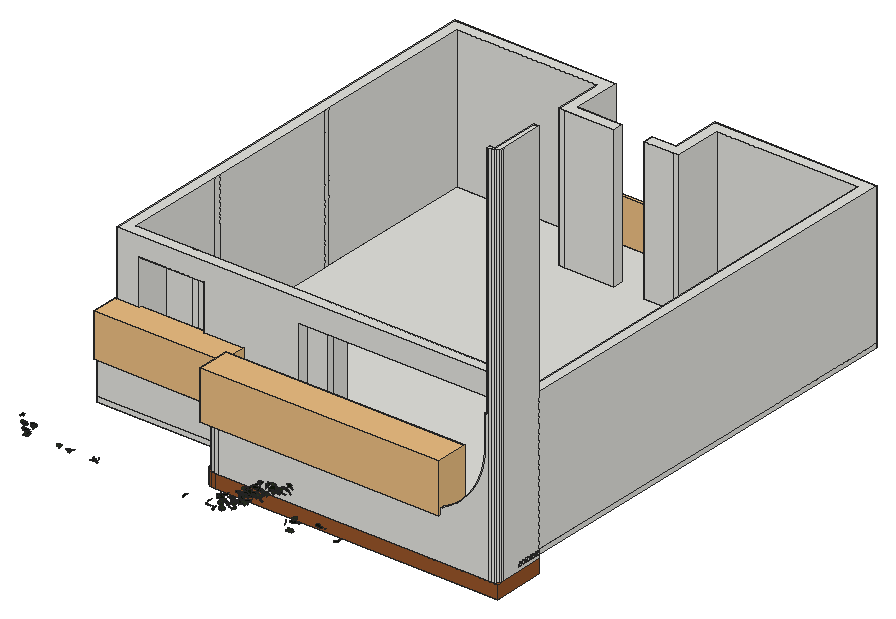
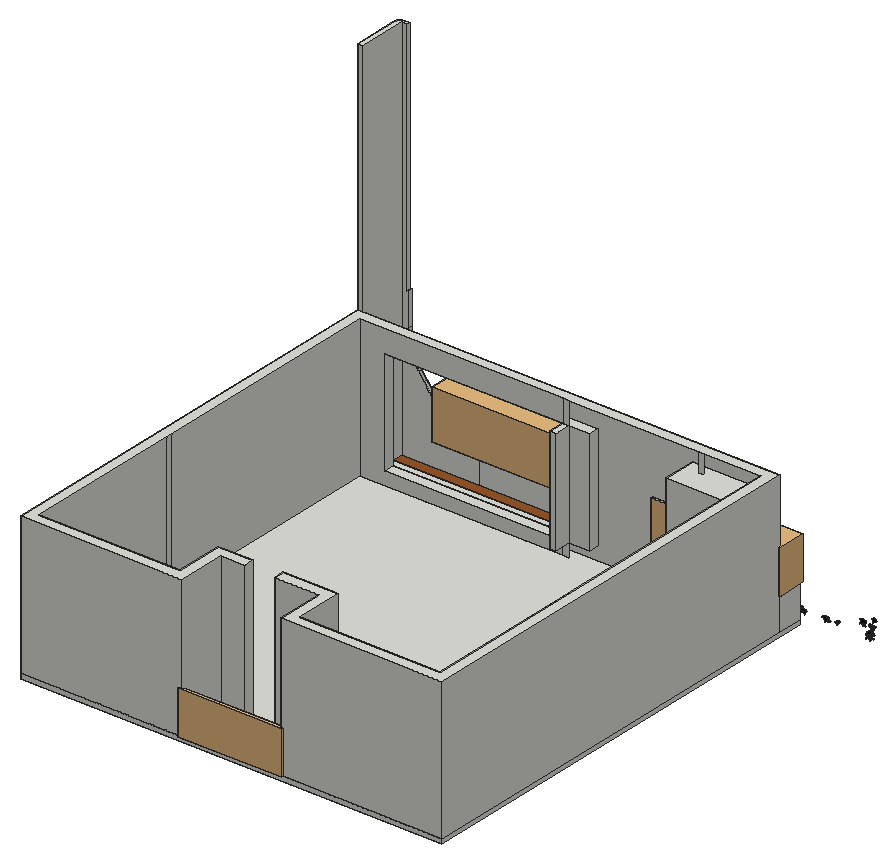
# SketchUp Ruby script. Lengths in millimetres.
U = 1.mm
M = Sketchup.active_model
def pt(a) = Geom::Point3d.new(a.map { |v| v * U })
def face(e, loops, mat)
  f = e.add_face(loops[0].map { |a| pt(a) })
  loops[1..].each { |l| e.add_face(l.map { |a| pt(a) }).erase! }
  f.material = f.back_material = mat if mat
  f
end
# faces: each face lists its corners as indices into pts; further lists are holes
def faces(e, pts, list, mat = nil) = list.each { |f| face(e, (f[0].is_a?(Array) ? f : [f]).map { |l| l.map { |i| pts[i] } }, mat) }
# xy, xz, yz: faces in a plane at the given z, y or x. An outline is a flat list of corners, or four numbers for a rectangle; further outlines are holes
def ring(l) = l.size == 4 ? [[l[0], l[1]], [l[2], l[1]], [l[2], l[3]], [l[0], l[3]]] : l.each_slice(2).to_a
def flat(e, list, mat, &to3) = list.each { |f| face(e, (f[0].is_a?(Array) ? f : [f]).map { |l| ring(l).map { |u, v| to3.(u, v) } }, mat) }
def xy(e, z, list, mat = nil) = flat(e, list, mat) { |x, y| [x, y, z] }
def xz(e, y, list, mat = nil) = flat(e, list, mat) { |x, z| [x, y, z] }
def yz(e, x, list, mat = nil) = flat(e, list, mat) { |y, z| [x, y, z] }
def lines(e, pts, list) = list.each { |a, b| e.add_line(pt(pts[a]), pt(pts[b])) }
# prism: a flat outline (further loops are holes) pulled along v
def prism(e, loops, v, mat = nil)
  f = face(e, loops, mat); d = Geom::Vector3d.new(v.map { |x| x * U })
  f.pushpull(f.normal.samedirection?(d) ? d.length : -d.length)
end
def box(e, o, s, mat = nil) = prism(e, [[o, [o[0] + s[0], o[1], o[2]], [o[0] + s[0], o[1] + s[1], o[2]], [o[0], o[1] + s[1], o[2]]]], [0, 0, s[2]], mat)
def at(x, y, z, deg = 0) = Geom::Transformation.translation(pt([x, y, z])) * Geom::Transformation.rotation(ORIGIN, Z_AXIS, deg.degrees)
def axes(o, x, y, z) = Geom::Transformation.new([*x, 0, *y, 0, *z, 0, *pt(o).to_a, 1])
def part(name) = M.definitions.add(name)
# library, detail: a bought-in or finely detailed component or shape, given as its bounding box
def library(name, o, s) = part(name).tap { |d| box(d.entities, o, s) }
def detail(e, o, s) = box(e.add_group.entities, o, s)
def put(e, d, t, mat = nil) = e.add_instance(d, t).tap { |i| i.material = mat if mat }
def group(e, t, mat = nil) = e.add_group.tap { |g| g.transformation = t; g.material = mat if mat }.entities
root = M.entities
M.materials.add("Emissive").color = [255, 185, 108]
M.materials.add("[Wood Cherry Original]").color = [152, 86, 42]
M.materials.add("efeu1").color = [18, 25, 13]
M.materials.add("efeu2").color = [43, 57, 29]
c1 = part("ivyleaf_10")
p = [[0,12.8,-0.8],[-1.5,51.3,-10.9],[-4.9,51,-11.6],[-13.6,26.5,-7.3],[-13.2,15.9,-4.6],[-21.1,19.3,-7.2],
  [-29.5,16.3,-8.3],[-29.2,8.3,-6.2],[-19.7,-9.8,0.5],[-7.6,-13,4],[1,-12.2,5.8],[-0.4,51.1,-11.1],
  [-1.5,51.1,-10.9],[1,-12.4,5.9],[16.9,-12.4,3.5],[35.1,9.1,-5.1],[35,12.9,-6.1],[20.5,16.4,-4.9],
  [15.8,15,-3.8],[15.3,27.6,-7.1],[12.8,31.3,-7.8]]
faces(c1.entities,p,[[0,1,2,3,4,5,6,7,8,9,10],[11,12,0,13,14,15,16,17,18,19,20]],"efeu2")
c2 = part("ivyleaf_9")
p = [[39.1,54.8,31.7],[34.5,51.8,30.2],[-5.3,25.2,17.3],[-17.9,28.3,20.9],[-21.6,21.7,17],[-20.2,4.3,5.3],
  [-22.9,-0.3,2.5],[-17.1,-4,-0.6],[-2,-2.1,-1.2],[-0.7,-15.4,-10.1],[16.6,-22.3,-16.7],[21.1,-15.1,-12.5],
  [32.7,-10.7,-11],[46.1,-1.8,-6.6],[30.8,11.2,3.8]]
faces(c2.entities,p,[[0,1,2,3,4,5,6,7,8,9,10,11,12,13,14]],"efeu1")
c3 = library("Group\#17",[0,0,0],[2782,637.9,939.4])
c4 = library("Group\#15",[0,0,0],[5171.1,707.5,1057.5])
c5 = part("Group\#8")
g1 = group(c5.entities,at(0,0,0))
xy(g1,0,[[0,0,0,9144,3500.3,9144,3500.3,8102.6,4459.1,8102.6,4459.1,7874,3276.6,7874,3276.6,8915.4,228.6,8915.4,228.6,228.6,8915.4,228.6,8915.4,8915.4,5867.4,8915.4,5867.4,7874,5119.1,7874,5119.1,8102.6,5638.8,8102.6,5638.8,9144,9144,9144,9144,0]])
xy(g1,288,[[3929.6,0,8374.6,228.6],[4394.2,228.6,4521.2,579.4]])
xy(g1,376.3,[[475.3,0,1877,723.9]])
xy(g1,2564.5,[[3929.6,0,8374.6,228.6],[4394.2,228.6,4521.2,579.4]])
xy(g1,2644.4,[[475.3,0,1877,723.9]])
xy(g1,3048,[[0,0,9144,0,9144,9144,5638.8,9144,5638.8,8102.6,5119.1,8102.6,5119.1,7874,5867.4,7874,5867.4,8915.4,8915.4,8915.4,8915.4,228.6,228.6,228.6,228.6,8915.4,3276.6,8915.4,3276.6,7874,4459.1,7874,4459.1,8102.6,3500.3,8102.6,3500.3,9144,0,9144]])
xz(g1,0,[[[0,0,9144,3048],[3929.6,288,8374.6,2564.5],[475.3,376.3,1877,2644.4]]])
xz(g1,228.6,[[1447.8,0,1574.8,3048],[4394.2,0,4521.2,288],[4521.2,0,4521.2,288,8374.6,288,8374.6,2564.5,4521.2,2564.5,4521.2,3048,8915.4,3048,8915.4,0],[3929.6,288,4394.2,2564.5],[4394.2,2564.5,4521.2,3048]])
xz(g1,579.4,[[4394.2,288,4521.2,2564.5]])
xz(g1,723.9,[[475.3,376.3,1877,2644.4]])
xz(g1,7874,[[3276.6,0,3403.6,3048],[3403.6,0,4459.1,3048],[5119.1,0,5740.4,3048],[5740.4,0,5867.4,3048]])
xz(g1,8102.6,[[3500.3,0,4459.1,3048],[5119.1,0,5638.8,3048]])
xz(g1,8915.4,[[228.6,0,3276.6,3048],[5867.4,0,8915.4,3048]])
xz(g1,9144,[[0,0,3500.3,3048],[5638.8,0,9144,3048]])
yz(g1,0,[[0,0,9144,3048]])
yz(g1,228.6,[[228.6,0,2362.2,3048],[2362.2,0,2489.2,3048],[2489.2,0,5334,3048],[5334,0,5461,3048],[5461,0,8915.4,3048]])
yz(g1,475.3,[[0,376.3,723.9,2644.4]])
yz(g1,1877,[[0,376.3,723.9,2644.4]])
yz(g1,3276.6,[[7874,0,8915.4,3048]])
yz(g1,3500.3,[[8102.6,0,9144,3048]])
yz(g1,3929.6,[[0,288,228.6,2564.5]])
yz(g1,4394.2,[[228.6,288,579.4,2564.5]])
yz(g1,4459.1,[[7874,0,8102.6,3048]])
yz(g1,4521.2,[[228.6,288,579.4,2564.5]])
yz(g1,5119.1,[[7874,0,8102.6,3048]])
yz(g1,5638.8,[[8102.6,0,9144,3048]])
yz(g1,5867.4,[[7874,0,8915.4,3048]])
yz(g1,8374.6,[[0,288,228.6,2564.5]])
yz(g1,8915.4,[[228.6,0,5334,3048],[5334,0,5461,3048],[5461,0,8915.4,3048]])
yz(g1,9144,[[0,0,9144,3048]])
c6 = library("Group\#25",[0,0,0],[2238.5,80,939.4])
p = [[1860.6,2460,2644.4],[3261.9,2460,2644.4],[10529.3,1836.4,3149.6],[10398.2,1836.4,3149.6],[10398.2,2446,3149.6],[10529.3,2446,3149.6]]
lines(root,p,[[0,1],[2,3],[4,5]])
put(root,c1,axes([2242.1,873.4,2679.7],[0.29759,-0.97706,-0.24122],[-0.00358,0.24383,-0.98885],[1.91537,0.15226,0.03563]))
put(root,c1,axes([4967.5,859.2,2851.4],[0.50779,0.74564,0.68177],[-0.36504,0.7297,-0.72299],[-1.8879,0.05946,0.32317]))
put(root,c1,axes([2158.9,869.8,2662.5],[-1.58433,0.57744,0.12979],[-0.21128,0.06767,-1.01309],[-1.1064,-0.83979,0.00761]))
put(root,c2,axes([5728.2,895.5,3110.4],[-0.3541,-0.44322,0.99252],[0.43909,-1.00012,-0.40336],[2.02162,0.13959,0.26145]))
put(root,c2,axes([5469.1,858,3018.6],[1.35654,0.76299,0.25695],[0.31308,0.19791,-1.04402],[-1.49993,0.73136,0.01446]))
put(root,c2,axes([724.9,864.8,2660.9],[0.00599,1.02644,-0.04252],[-0.00314,-0.0425,-1.02645],[-1.25332,0.00501,0.00236]))
put(root,c1,axes([684,878,2636.9],[1.19057,0.38067,-0.02341],[-0.02529,-0.01128,-1.04749],[-0.46461,0.97609,-0.00297]))
put(root,c1,axes([1610.6,870,2612.4],[0.34837,-0.0135,1.0075],[-1.8784,0.20373,0.18204],[-0.38602,-1.00352,0.02341]))
put(root,c1,axes([691.1,871.7,2819.8],[-0.60714,0.25021,-0.8928],[-0.93426,0.46035,0.55588],[0.63775,0.91259,-0.03563]))
put(root,c2,axes([4591,877.2,2635.9],[1.62005,-0.33682,0.41046],[0.77692,-0.08081,-0.91287],[0.64621,0.94156,0.06849]))
put(root,c2,axes([4099,856,2629.3],[0.55858,0.36321,1.03584],[1.02656,0.88612,-0.46354],[-1.81947,0.61146,0.05647]))
put(root,c1,axes([1376.7,875.6,2657.5],[1.27455,0.75499,0.11689],[-0.11631,0.20788,-0.99257],[-1.44935,0.64725,0.18245]))
put(root,c1,axes([595.4,883.2,2836.8],[1.06507,0.56369,-0.10968],[-0.10229,-0.07232,-1.03907],[-0.69309,0.87689,-0.01519]))
put(root,c2,axes([1630.6,865.8,2650.6],[1.18403,0.82066,-0.01773],[-0.22401,0.06716,-1.02102],[-1.54611,0.61874,0.13435]))
put(root,c2,axes([809.8,872.9,2874.2],[1.94041,0.16715,-0.03853],[-0.0612,-0.04191,-1.03253],[-0.32068,1.01942,-0.03613]))
put(root,c2,axes([626.5,868.6,2820.3],[1.01133,0.62198,-0.21562],[-0.30144,-0.0274,-1.02894],[-0.7444,0.85611,0.12372]))
put(root,c2,axes([2122.5,870.6,2617.5],[1.93414,0.05111,0.00473],[-0.01003,0.19729,-0.99823],[-0.09717,0.99693,0.1973]))
put(root,c1,axes([4923.3,889.9,2680.2],[1.09544,0.55557,-0.6352],[-0.98394,-0.37555,-0.79693],[-1.26938,0.77054,0.06957]))
put(root,c2,axes([666.7,888.3,2634.2],[-1.20615,0.2778,-0.01695],[0.00023,-0.06187,-1.02521],[-0.33955,-0.98685,0.05951]))
put(root,c2,axes([583.4,867.1,2972.5],[0.68149,0.89293,0.21313],[0.1496,0.17468,-1.0532],[-1.10994,0.57179,-0.01109]))
put(root,c2,axes([6980,884.2,3058.4],[0.79399,0.16085,-1.15793],[2.00309,0.48349,0.44636],[0.96848,-1.13185,0.02611]))
put(root,c2,axes([2108.7,872.1,2628.9],[0.38033,0.98848,0.13533],[-0.0569,0.14388,-1.00685],[-1.89798,0.19376,0.0573]))
put(root,c2,axes([654.6,871.8,2705.4],[1.00699,0.3655,0.52651],[0.55106,0.27736,-0.90063],[-0.55478,0.93892,0.06109]))
put(root,c2,axes([5332.8,887.7,2945.9],[-0.4729,-0.71957,-0.74613],[0.55117,0.68852,-0.76046],[1.89426,-0.37998,0.035]))
put(root,c1,axes([827.3,880,2813.5],[0.68505,-0.31545,-0.90782],[-1.32482,0.58282,-0.47852],[1.26115,0.7836,-0.00955]))
put(root,c1,axes([614,890.3,2761],[0.32792,-0.99845,-0.0849],[-0.04066,0.07894,-1.03393],[1.22183,0.2706,-0.01162]))
put(root,c1,axes([5409.5,893.3,2948.9],[2.01643,-0.11215,-0.11915],[-0.22506,0.01476,-1.06541],[0.21524,1.06607,0.00222]))
put(root,c2,axes([4719.6,879.5,2604.8],[0.15912,0.02228,-1.00472],[-1.7006,0.46305,-0.06409],[0.87533,0.89557,0.05813]))
put(root,c1,axes([610.5,895.2,2693.7],[-1.21188,-0.22111,0.05207],[-0.05777,-0.02687,-1.01754],[0.27105,-0.99435,0.01591]))
put(root,c1,axes([6293.6,880.7,2880],[0.29531,-0.72314,-1.01067],[-0.35276,0.99366,-0.73943],[2.33871,0.24119,0.01609]))
put(root,c1,axes([4877.8,895.9,2644.8],[1.73286,0.40859,0.19804],[0.28431,0.14949,-0.99524],[-0.81604,0.91972,0.07378]))
put(root,c2,axes([651.5,894.1,2658.9],[1.23921,-0.1475,-0.04468],[-0.05298,0.01185,-1.02638],[0.1804,1.01666,0.00548]))
put(root,c1,axes([686.9,895.7,2656.7],[0.6209,0.83618,0.3194],[0.1711,0.28839,-0.97846],[-1.07854,0.52712,0.02865]))
put(root,c2,axes([711.3,906,2616.1],[-1.11801,0.34409,0.24843],[-0.2952,0.06208,-0.97852],[-0.42538,-0.94745,0.02611]))
put(root,c1,axes([661.3,885.6,2591],[-0.01799,0.45905,-0.93566],[0.02275,0.93572,0.45878],[1.27128,-0.01025,-0.02145]))
put(root,c2,axes([4737.8,890.4,2611.3],[-0.17432,0.95753,0.30224],[-0.07245,0.29996,-0.96186],[-1.90962,-0.09879,0.0089]))
put(root,c1,axes([6459,887,3011.5],[0.43261,0.68832,0.95487],[0.34183,0.94084,-0.72096],[-2.21401,0.27975,0.07527]))
put(root,c2,axes([696.6,888.8,2641.7],[0.73939,0.77669,0.281],[0.16249,0.25207,-0.98399],[-0.99448,0.61865,0.04815]))
put(root,c2,axes([6416,895.1,2928.2],[1.83795,0.2001,0.67518],[1.25058,0.15607,-0.9861],[-0.48199,1.16796,0.01609]))
put(root,c1,axes([5158.9,923.7,2746.8],[0.06803,0.74348,-0.73897],[-1.07018,-0.61042,-0.64135],[-1.68372,0.41802,0.37778]))
put(root,c1,axes([6374,929.2,2723.5],[1.02772,0.08734,-1.12827],[-2.12441,-0.1645,-0.54697],[-0.35423,1.23997,0.00691]))
put(root,c1,axes([626.7,907.5,2629.8],[0.08799,0.56648,0.83577],[-0.5279,0.77439,-0.48754],[-1.11293,-0.32253,0.29733]))
put(root,c2,axes([7360.5,914,2874.3],[0.99165,1.17741,0.39801],[0.30308,0.36477,-1.28755],[-2.34592,0.54483,0.0019]))
put(root,c2,axes([5096.3,1016.4,2816.7],[1.61558,-0.4369,-0.43493],[-0.67908,0.25539,-0.95294],[0.95679,0.91899,0.05806]))
put(root,c2,axes([5354.1,1034.3,3117.3],[-0.98874,-0.36875,-0.89917],[1.67357,0.25577,-0.61295],[0.78754,-1.00647,0.17367]))
put(root,c2,axes([5931.6,1031.2,3365.2],[-1.98819,0.52194,0.01236],[-0.02445,0.00195,-1.16778],[-0.99334,-1.04473,0.004]))
put(root,c2,axes([5387.1,1037,3161.5],[-1.30777,0.56503,-0.61847],[0.72498,-0.50168,-0.88156],[-1.41997,-0.77652,0.11951]))
put(root,c2,axes([5298.2,1018.6,3047.3],[1.5576,0.68968,-0.24282],[-0.37984,-0.1399,-1.07006],[-1.33874,0.84213,0.0211]))
put(root,c2,axes([5616.5,1025,3357.9],[1.76921,-0.04931,0.62228],[1.18679,0.12456,-0.92166],[-0.05451,1.1117,0.13087]))
put(root,c2,axes([5493.5,1032.3,3222],[1.0405,0.65027,-0.69072],[-0.97441,-0.46888,-0.84667],[-1.51996,0.74574,0.06995]))
put(root,c1,axes([5249.1,1042.8,3113.7],[0.64652,1.01263,-0.20331],[-0.17538,-0.18345,-1.06771],[-1.95787,0.35082,0.02851]))
put(root,c1,axes([5602.3,1031,3339],[-0.30681,1.04009,0.36399],[-0.09139,0.36088,-1.05249],[-2.09523,-0.16804,-0.00739]))
put(root,c2,axes([5518.4,1027.3,3267.7],[0.90088,0.98786,0.11357],[0.06997,0.10831,-1.09532],[-1.89118,0.47458,0.01358]))
put(root,c2,axes([4778.7,1052.3,2770.1],[-1.94504,0.12001,0.16733],[-0.3162,0.01988,-1.02901],[-0.23152,-1.0354,-0.00036]))
put(root,c2,axes([5199.6,1054.3,2899.6],[1.00746,-0.95965,0.0234],[0.04472,-0.01376,-1.09588],[1.8264,0.52969,0.01393]))
put(root,c1,axes([5145.5,1048.6,2992.1],[0.69393,0.97253,-0.19472],[-0.23672,-0.16099,-1.03696],[-1.87275,0.38071,0.05892]))
put(root,c1,axes([6035.4,1046.8,3358.8],[-1.56865,-0.81256,-0.11223],[0.195,0.05587,-1.15696],[1.54891,-0.82994,0.03199]))
put(root,c1,axes([6012.2,1053.4,3344.1],[-0.6475,-1.1092,0.03978],[0.68741,-0.14998,-1.09302],[1.9974,-0.30795,0.38906]))
put(root,c1,axes([5732.1,1051.9,3170.1],[2.0977,-0.07402,0.25396],[0.49824,0.14926,-1.0927],[0.07216,1.12118,0.16224]))
put(root,c2,axes([5578.6,1058.5,3196.6],[-1.20779,0.6911,-0.64158],[0.80648,-0.48186,-0.9382],[-1.6033,-0.763,0.01139]))
put(root,c2,axes([4756.1,1049.5,2783.6],[-0.7255,0.91992,-0.26859],[0.15775,-0.25632,-0.99556],[-1.81705,-0.38955,0.02081]))
put(root,c1,axes([5905.9,1055.8,3388.3],[2.00327,-0.33927,-0.20892],[-0.36497,0.08593,-1.10567],[0.6647,1.06967,0.02256]))
put(root,c1,axes([5654.4,1055.3,3191.2],[1.20275,-0.88658,-0.11473],[0.06846,0.1656,-1.0816],[1.70004,0.62057,0.12472]))
put(root,c1,axes([5579,1056.1,3074.9],[1.98723,-0.0017,0.4011],[0.75385,0.18066,-1.03034],[-0.12031,1.10386,0.16924]))
put(root,c2,axes([4850.7,1051.6,2714.5],[1.25281,0.26493,-0.7795],[-1.39844,-0.26112,-0.70925],[-0.70676,0.98628,0.02161]))
put(root,c2,axes([5115.2,1046.6,2980.6],[1.57089,0.01301,0.69398],[1.26714,0.28996,-0.79731],[-0.37342,1.03866,0.21388]))
put(root,c1,axes([4738.1,1072.3,2657.9],[0.68708,0.55538,-0.76273],[-0.9381,-0.58534,-0.65952],[-1.53116,0.60784,0.06181]))
put(root,c1,axes([5712.2,1063.4,3165.4],[-0.17705,-1.12959,-0.04249],[0.05199,0.04038,-1.13316],[2.15072,-0.09397,0.02389]))
put(root,c1,axes([5241.4,1067.2,2980.7],[-1.50802,0.42248,-0.63949],[0.9626,-0.40287,-0.89284],[-1.096,-0.93514,0.09573]))
put(root,c1,axes([5271.5,1068.8,2956.3],[-0.01799,-1.05869,0.08056],[0.05869,-0.0808,-1.05826],[2.01987,-0.00708,0.03147]))
put(root,c1,axes([4739.7,1060.1,2618.7],[-1.89903,0.13306,0.2763],[-0.51695,0.05316,-1.00651],[-0.27096,-1.03399,-0.01619]))
put(root,c2,axes([4728.5,1053.6,2761.5],[-0.66833,0.80842,0.52756],[-0.49945,0.4603,-0.88003],[-1.76804,-0.43562,0.04917]))
put(root,c2,axes([4722.9,1058.2,2741.6],[1.38605,0.40307,-0.59217],[-1.12846,-0.13467,-0.82086],[-0.76502,0.92893,0.13795]))
put(root,c1,axes([5935.1,1068.6,3269.4],[1.24034,-0.07385,0.94765],[1.80339,0.14119,-0.64064],[-0.14283,1.14142,0.14056]))
put(root,c2,axes([5275.8,1060.8,2974.8],[1.78278,-0.1931,-0.46559],[-0.83018,0.18181,-0.953],[0.48071,1.03014,0.08091]))
put(root,c2,axes([5166.2,1073.6,2909.5],[0.37753,-0.94925,-0.41107],[0.15478,0.43158,-0.95735],[1.96264,0.14856,0.15457]))
put(root,c2,axes([6152.4,1080.9,3377.4],[1.15246,-0.99144,0.14789],[0.18487,-0.11393,-1.1615],[1.89881,0.61284,0.02332]))
put(root,c2,axes([5310.5,1071.8,3007.9],[-0.15698,-0.22134,-1.041],[1.60289,0.62477,-0.19957],[1.23835,-0.83675,0.12636]))
put(root,c1,axes([5157.7,1074.1,2817.4],[0.90985,-0.96265,-0.08008],[0.31675,0.1701,-1.0512],[1.81095,0.4539,0.22409]))
put(root,c1,axes([5734.3,1069.3,3288.7],[0.59861,-0.97288,-0.4263],[-0.22162,0.41034,-1.02236],[2.00936,0.33509,0.01424]))
put(root,c1,axes([4997.6,1074.3,2770.1],[-0.88592,-0.91247,-0.12137],[0.43309,0.01771,-1.00594],[1.69753,-0.48073,0.19331]))
put(root,c1,axes([4960,1074.4,2816.4],[-1.36327,-0.74428,0.00579],[-0.00611,-0.00494,-1.03298],[1.41655,-0.71631,0.00111]))
put(root,c2,axes([4502.1,1063.3,2600.4],[-0.15659,0.99517,0.0254],[-0.06349,0.02271,-0.99807],[-1.89356,-0.08306,0.03136]))
put(root,c2,axes([5777,1053.6,3338.6],[0.22454,0.63617,0.90572],[-0.36519,0.90882,-0.61334],[-2.07459,-0.09112,0.20599]))
put(root,c1,axes([4973.2,1072.8,2797.9],[0.07438,1.03091,0.06279],[-0.00467,0.06293,-1.03164],[-1.96566,0.03886,0.00483]))
put(root,c2,axes([4823.4,1057.2,2828.6],[1.16542,0.69984,0.47488],[0.46449,0.41513,-0.92648],[-1.54116,0.65433,0.07987]))
put(root,c1,axes([5873.9,1074.8,3257.7],[-1.87612,0.38988,0.45301],[-0.95555,-0.06614,-1.03562],[-0.61712,-1.08286,0.22635]))
put(root,c2,axes([5442,1063.6,3075],[1.76945,0.54423,0.06894],[0.07148,0.07219,-1.07643],[-1.04161,0.92948,0.04324]))
put(root,c2,axes([4854,1076,2639.1],[1.67937,-0.51416,-0.24126],[-0.2851,0.21927,-1.01521],[1.04264,0.88811,0.11099]))
put(root,c1,axes([4978.9,1078.8,2782.2],[-1.47353,0.67422,0.12444],[-0.37453,-0.03873,-1.01453],[-1.24994,-0.78322,0.15729]))
put(root,c1,axes([4992.7,1079.7,2710.3],[-1.80108,0.43212,0.20093],[-0.3777,0.04881,-1.03966],[-0.82458,-0.96621,0.03734]))
put(root,c2,axes([5608.9,1110.8,3107.8],[-0.49555,-0.71974,0.82282],[0.18275,-0.85762,-0.7198],[2.07251,-0.09647,0.26021]))
put(root,c1,axes([5469.8,1086.7,3019.5],[-1.99649,-0.30508,-0.21695],[0.43862,-0.01764,-1.08956],[0.56145,-1.07107,0.07974]))
put(root,c1,axes([5452.7,1094.3,3000.8],[-1.3568,0.81841,-0.22686],[0.27371,-0.17558,-1.08535],[-1.593,-0.72724,0.00674]))
put(root,c1,axes([5053.8,1098.1,2759.4],[1.80273,0.36869,-0.33995],[-0.66553,-0.03519,-1.01251],[-0.68413,1.00575,0.08919]))
put(root,c2,axes([5956.1,1089.7,3255.1],[1.77598,0.05882,0.67245],[1.276,0.05245,-0.93497],[-0.14916,1.14901,0.00825]))
put(root,c1,axes([5183.8,1102.4,2783.9],[1.47497,-0.71395,-0.2171],[-0.34001,0.12638,-1.05337],[1.37893,0.79484,-0.02752]))
put(root,c2,axes([6181.3,1109.2,3466.2],[0.7666,-1.07979,-0.23813],[-0.12373,0.22987,-1.15231],[2.10079,0.40756,0.01903]))
put(root,c2,axes([5815.1,1109.6,3247.7],[-0.46848,-1.0055,-0.48905],[0.22168,0.47498,-1.03519],[2.11643,-0.27232,0.00017]))
put(root,c2,axes([6064.7,1108.1,3368.3],[2.01851,-0.47378,0.069],[0.11377,-0.03535,-1.16157],[0.90407,1.06224,-0.00788]))
put(root,c1,axes([4949.5,1119.2,2688.5],[-1.5966,-0.40827,-0.49554],[1.01279,0.01408,-0.91248],[0.68373,-0.97423,0.19448]))
put(root,c2,axes([4874.9,1132.3,2633.6],[1.63187,0.58964,0.10067],[0.10232,0.09927,-1.03936],[-1.13384,0.8576,0.0511]))
g2 = group(root,at(4151.8,1531.6,2669.4),"[Wood Cherry Original]")
xy(g2,0,[[[6377.5,-209.6,265.9,-209.5,184.6,-202.2,118.2,-180,66.5,-143.1,29.5,-91.4,7.4,-24.9,0,56.3,0,914.4,6377.5,914.4],[4138.7,109.7,4197.4,117.4,4252.2,140.1,4299.2,176.2,4335.3,223.2,4357.9,278,4365.7,336.7,4357.9,395.5,4335.3,450.2,4299.2,497.2,4252.2,533.3,4197.4,556,4138.7,563.7,4079.9,556,4025.1,533.3,3978.1,497.2,3942.1,450.2,3919.4,395.5,3911.6,336.7,3919.4,278,3942.1,223.2,3978.1,176.2,4025.1,140.1,4079.9,117.4],[2346.9,109.7,2405.7,117.4,2460.4,140.1,2507.4,176.2,2543.5,223.2,2566.2,278,2573.9,336.7,2566.2,395.5,2543.5,450.2,2507.4,497.2,2460.4,533.3,2405.7,556,2346.9,563.7,2288.1,556,2233.4,533.3,2186.4,497.2,2150.3,450.2,2127.6,395.5,2119.9,336.7,2127.6,278,2150.3,223.2,2186.4,176.2,2233.4,140.1,2288.1,117.4],[555.1,109.7,613.9,117.4,668.6,140.1,715.7,176.2,751.7,223.2,774.4,278,782.1,336.7,774.4,395.5,751.7,450.2,715.7,497.2,668.6,533.3,613.9,556,555.1,563.7,496.4,556,441.6,533.3,394.6,497.2,358.5,450.2,335.9,395.5,328.1,336.7,335.9,278,358.5,223.2,394.6,176.2,441.6,140.1,496.4,117.4],[5930.4,109.7,5989.2,117.4,6043.9,140.1,6090.9,176.2,6127,223.2,6149.7,278,6157.4,336.7,6149.7,395.5,6127,450.2,6090.9,497.2,6043.9,533.3,5989.2,556,5930.4,563.7,5871.7,556,5816.9,533.3,5769.9,497.2,5733.8,450.2,5711.1,395.5,5703.4,336.7,5711.1,278,5733.8,223.2,5769.9,176.2,5816.9,140.1,5871.7,117.4]],[[555.1,109.7,496.4,117.4,441.6,140.1,394.6,176.2,358.5,223.2,335.9,278,328.1,336.7,335.9,395.5,358.5,450.2,394.6,497.2,441.6,533.3,496.4,556,555.1,563.7,613.9,556,668.6,533.3,715.7,497.2,751.7,450.2,774.4,395.5,782.1,336.7,774.4,278,751.7,223.2,715.7,176.2,668.6,140.1,613.9,117.4],[555.1,166.8,599.1,172.6,640.1,189.6,675.2,216.6,702.2,251.8,719.2,292.7,725,336.7,719.2,380.7,702.2,421.6,675.2,456.8,640.1,483.8,599.1,500.8,555.1,506.6,511.2,500.8,470.2,483.8,435,456.8,408,421.6,391.1,380.7,385.3,336.7,391.1,292.7,408,251.8,435,216.6,470.2,189.6,511.2,172.6]],[[2346.9,109.7,2288.1,117.4,2233.4,140.1,2186.4,176.2,2150.3,223.2,2127.6,278,2119.9,336.7,2127.6,395.5,2150.3,450.2,2186.4,497.2,2233.4,533.3,2288.1,556,2346.9,563.7,2405.7,556,2460.4,533.3,2507.4,497.2,2543.5,450.2,2566.2,395.5,2573.9,336.7,2566.2,278,2543.5,223.2,2507.4,176.2,2460.4,140.1,2405.7,117.4],[2346.9,166.8,2390.9,172.6,2431.8,189.6,2467,216.6,2494,251.8,2511,292.7,2516.8,336.7,2511,380.7,2494,421.6,2467,456.8,2431.8,483.8,2390.9,500.8,2346.9,506.6,2302.9,500.8,2262,483.8,2226.8,456.8,2199.8,421.6,2182.8,380.7,2177,336.7,2182.8,292.7,2199.8,251.8,2226.8,216.6,2262,189.6,2302.9,172.6]],[[4138.7,109.7,4079.9,117.4,4025.1,140.1,3978.1,176.2,3942.1,223.2,3919.4,278,3911.6,336.7,3919.4,395.5,3942.1,450.2,3978.1,497.2,4025.1,533.3,4079.9,556,4138.7,563.7,4197.4,556,4252.2,533.3,4299.2,497.2,4335.3,450.2,4357.9,395.5,4365.7,336.7,4357.9,278,4335.3,223.2,4299.2,176.2,4252.2,140.1,4197.4,117.4],[4138.7,166.8,4182.6,172.6,4223.6,189.6,4258.8,216.6,4285.8,251.8,4302.7,292.7,4308.5,336.7,4302.7,380.7,4285.8,421.6,4258.8,456.8,4223.6,483.8,4182.6,500.8,4138.7,506.6,4094.7,500.8,4053.7,483.8,4018.5,456.8,3991.5,421.6,3974.6,380.7,3968.8,336.7,3974.6,292.7,3991.5,251.8,4018.5,216.6,4053.7,189.6,4094.7,172.6]],[[5930.4,109.7,5871.7,117.4,5816.9,140.1,5769.9,176.2,5733.8,223.2,5711.1,278,5703.4,336.7,5711.1,395.5,5733.8,450.2,5769.9,497.2,5816.9,533.3,5871.7,556,5930.4,563.7,5989.2,556,6043.9,533.3,6090.9,497.2,6127,450.2,6149.7,395.5,6157.4,336.7,6149.7,278,6127,223.2,6090.9,176.2,6043.9,140.1,5989.2,117.4],[5930.4,166.8,5974.4,172.6,6015.3,189.6,6050.5,216.6,6077.5,251.8,6094.5,292.7,6100.3,336.7,6094.5,380.7,6077.5,421.6,6050.5,456.8,6015.3,483.8,5974.4,500.8,5930.4,506.6,5886.4,500.8,5845.5,483.8,5810.3,456.8,5783.3,421.6,5766.3,380.7,5760.5,336.7,5766.3,292.7,5783.3,251.8,5810.3,216.6,5845.5,189.6,5886.4,172.6]]])
xy(g2,100,[[555.1,166.8,511.2,172.6,470.2,189.6,435,216.6,408,251.8,391.1,292.7,385.3,336.7,391.1,380.7,408,421.6,435,456.8,470.2,483.8,511.2,500.8,555.1,506.6,599.1,500.8,640.1,483.8,675.2,456.8,702.2,421.6,719.2,380.7,725,336.7,719.2,292.7,702.2,251.8,675.2,216.6,640.1,189.6,599.1,172.6]],"Emissive")
xy(g2,138.1,[[2346.9,166.8,2302.9,172.6,2262,189.6,2226.8,216.6,2199.8,251.8,2182.8,292.7,2177,336.7,2182.8,380.7,2199.8,421.6,2226.8,456.8,2262,483.8,2302.9,500.8,2346.9,506.6,2390.9,500.8,2431.8,483.8,2467,456.8,2494,421.6,2511,380.7,2516.8,336.7,2511,292.7,2494,251.8,2467,216.6,2431.8,189.6,2390.9,172.6],[4138.7,166.8,4094.7,172.6,4053.7,189.6,4018.5,216.6,3991.5,251.8,3974.6,292.7,3968.8,336.7,3974.6,380.7,3991.5,421.6,4018.5,456.8,4053.7,483.8,4094.7,500.8,4138.7,506.6,4182.6,500.8,4223.6,483.8,4258.8,456.8,4285.8,421.6,4302.7,380.7,4308.5,336.7,4302.7,292.7,4285.8,251.8,4258.8,216.6,4223.6,189.6,4182.6,172.6],[5930.4,166.8,5886.4,172.6,5845.5,189.6,5810.3,216.6,5783.3,251.8,5766.3,292.7,5760.5,336.7,5766.3,380.7,5783.3,421.6,5810.3,456.8,5845.5,483.8,5886.4,500.8,5930.4,506.6,5974.4,500.8,6015.3,483.8,6050.5,456.8,6077.5,421.6,6094.5,380.7,6100.3,336.7,6094.5,292.7,6077.5,251.8,6050.5,216.6,6015.3,189.6,5974.4,172.6]],"Emissive")
xy(g2,290.5,[[6377.5,-209.6,6377.5,914.4,0,914.4,0,56.3,7.4,-24.9,29.5,-91.4,66.5,-143.1,118.2,-180,184.6,-202.2,265.9,-209.5]])
xz(g2,914.4,[[0,0,6377.5,290.5]])
yz(g2,0,[[56.3,0,914.4,290.5]])
yz(g2,6377.5,[[-209.6,0,914.4,290.5]])
p = [[265.9,-209.5,0],[6377.5,-209.6,0],[6377.5,-209.6,290.5],[265.9,-209.5,290.5],[184.6,-202.2,290.5],[184.6,-202.2,0],
  [118.2,-180,290.5],[118.2,-180,0],[66.5,-143.1,290.5],[66.5,-143.1,0],[29.5,-91.4,290.5],[29.5,-91.4,0],
  [7.4,-24.9,290.5],[7.4,-24.9,0],[0,56.3,290.5],[0,56.3,0],[555.1,166.8,0],[511.2,172.6,0],
  [511.2,172.6,100],[555.1,166.8,100],[599.1,172.6,0],[599.1,172.6,100],[2346.9,166.8,0],[2302.9,172.6,0],
  [2302.9,172.6,138.1],[2346.9,166.8,138.1],[2390.9,172.6,0],[2390.9,172.6,138.1],[4138.7,166.8,0],[4094.7,172.6,0],
  [4094.7,172.6,138.1],[4138.7,166.8,138.1],[4182.6,172.6,0],[4182.6,172.6,138.1],[5930.4,166.8,0],[5886.4,172.6,0],
  [5886.4,172.6,138.1],[5930.4,166.8,138.1],[5974.4,172.6,0],[5974.4,172.6,138.1],[470.2,189.6,0],[470.2,189.6,100],
  [640.1,189.6,0],[640.1,189.6,100],[2262,189.6,0],[2262,189.6,138.1],[2431.8,189.6,0],[2431.8,189.6,138.1],
  [4053.7,189.6,0],[4053.7,189.6,138.1],[4223.6,189.6,0],[4223.6,189.6,138.1],[5845.5,189.6,0],[5845.5,189.6,138.1],
  [6015.3,189.6,0],[6015.3,189.6,138.1],[435,216.6,0],[435,216.6,100],[675.2,216.6,0],[675.2,216.6,100],
  [2226.8,216.6,0],[2226.8,216.6,138.1],[2467,216.6,0],[2467,216.6,138.1],[4018.5,216.6,0],[4018.5,216.6,138.1],
  [4258.8,216.6,0],[4258.8,216.6,138.1],[5810.3,216.6,0],[5810.3,216.6,138.1],[6050.5,216.6,0],[6050.5,216.6,138.1],
  [408,251.8,0],[408,251.8,100],[702.2,251.8,0],[702.2,251.8,100],[2199.8,251.8,0],[2199.8,251.8,138.1],
  [2494,251.8,0],[2494,251.8,138.1],[3991.5,251.8,0],[3991.5,251.8,138.1],[4285.8,251.8,0],[4285.8,251.8,138.1],
  [5783.3,251.8,0],[5783.3,251.8,138.1],[6077.5,251.8,0],[6077.5,251.8,138.1],[391.1,292.7,0],[391.1,292.7,100],
  [719.2,292.7,0],[719.2,292.7,100],[2182.8,292.7,0],[2182.8,292.7,138.1],[2511,292.7,0],[2511,292.7,138.1],
  [3974.6,292.7,0],[3974.6,292.7,138.1],[4302.7,292.7,0],[4302.7,292.7,138.1],[5766.3,292.7,0],[5766.3,292.7,138.1],
  [6094.5,292.7,0],[6094.5,292.7,138.1],[385.3,336.7,0],[385.3,336.7,100],[725,336.7,0],[725,336.7,100],
  [2177,336.7,0],[2177,336.7,138.1],[2516.8,336.7,0],[2516.8,336.7,138.1],[3968.8,336.7,0],[3968.8,336.7,138.1],
  [4308.5,336.7,0],[4308.5,336.7,138.1],[5760.5,336.7,0],[5760.5,336.7,138.1],[6100.3,336.7,0],[6100.3,336.7,138.1],
  [391.1,380.7,0],[391.1,380.7,100],[719.2,380.7,0],[719.2,380.7,100],[2182.8,380.7,0],[2182.8,380.7,138.1],
  [2511,380.7,0],[2511,380.7,138.1],[3974.6,380.7,0],[3974.6,380.7,138.1],[4302.7,380.7,0],[4302.7,380.7,138.1],
  [5766.3,380.7,0],[5766.3,380.7,138.1],[6094.5,380.7,0],[6094.5,380.7,138.1],[408,421.6,0],[408,421.6,100],
  [702.2,421.6,0],[702.2,421.6,100],[2199.8,421.6,0],[2199.8,421.6,138.1],[2494,421.6,0],[2494,421.6,138.1],
  [3991.5,421.6,0],[3991.5,421.6,138.1],[4285.8,421.6,0],[4285.8,421.6,138.1],[5783.3,421.6,0],[5783.3,421.6,138.1],
  [6077.5,421.6,0],[6077.5,421.6,138.1],[435,456.8,0],[435,456.8,100],[675.2,456.8,0],[675.2,456.8,100],
  [2226.8,456.8,0],[2226.8,456.8,138.1],[2467,456.8,0],[2467,456.8,138.1],[4018.5,456.8,0],[4018.5,456.8,138.1],
  [4258.8,456.8,0],[4258.8,456.8,138.1],[5810.3,456.8,0],[5810.3,456.8,138.1],[6050.5,456.8,0],[6050.5,456.8,138.1],
  [470.2,483.8,0],[470.2,483.8,100],[640.1,483.8,0],[640.1,483.8,100],[2262,483.8,0],[2262,483.8,138.1],
  [2431.8,483.8,0],[2431.8,483.8,138.1],[4053.7,483.8,0],[4053.7,483.8,138.1],[4223.6,483.8,0],[4223.6,483.8,138.1],
  [5845.5,483.8,0],[5845.5,483.8,138.1],[6015.3,483.8,0],[6015.3,483.8,138.1],[511.2,500.8,0],[511.2,500.8,100],
  [599.1,500.8,0],[599.1,500.8,100],[2302.9,500.8,0],[2302.9,500.8,138.1],[2390.9,500.8,0],[2390.9,500.8,138.1],
  [4094.7,500.8,0],[4094.7,500.8,138.1],[4182.6,500.8,0],[4182.6,500.8,138.1],[5886.4,500.8,0],[5886.4,500.8,138.1],
  [5974.4,500.8,0],[5974.4,500.8,138.1],[555.1,506.6,0],[555.1,506.6,100],[2346.9,506.6,0],[2346.9,506.6,138.1],
  [4138.7,506.6,0],[4138.7,506.6,138.1],[5930.4,506.6,0],[5930.4,506.6,138.1]]
faces(g2,p,[[0,1,2,3],[0,3,4,5],[5,4,6,7],[7,6,8,9],[9,8,10,11],[11,10,12,13],[13,12,14,15]])
faces(g2,p,[[16,17,18,19],[20,16,19,21],[22,23,24,25],[26,22,25,27],[28,29,30,31],[32,28,31,33],[34,35,36,37],[38,34,37,39],
  [17,40,41,18],[42,20,21,43],[23,44,45,24],[46,26,27,47],[29,48,49,30],[50,32,33,51],[35,52,53,36],[54,38,39,55],
  [40,56,57,41],[58,42,43,59],[44,60,61,45],[62,46,47,63],[48,64,65,49],[66,50,51,67],[52,68,69,53],[70,54,55,71],
  [56,72,73,57],[74,58,59,75],[60,76,77,61],[78,62,63,79],[64,80,81,65],[82,66,67,83],[68,84,85,69],[86,70,71,87],
  [72,88,89,73],[90,74,75,91],[76,92,93,77],[94,78,79,95],[80,96,97,81],[98,82,83,99],[84,100,101,85],[102,86,87,103],
  [88,104,105,89],[106,90,91,107],[92,108,109,93],[110,94,95,111],[96,112,113,97],[114,98,99,115],[100,116,117,101],[118,102,103,119],
  [104,120,121,105],[122,106,107,123],[108,124,125,109],[126,110,111,127],[112,128,129,113],[130,114,115,131],[116,132,133,117],[134,118,119,135],
  [120,136,137,121],[138,122,123,139],[124,140,141,125],[142,126,127,143],[128,144,145,129],[146,130,131,147],[132,148,149,133],[150,134,135,151],
  [136,152,153,137],[154,138,139,155],[140,156,157,141],[158,142,143,159],[144,160,161,145],[162,146,147,163],[148,164,165,149],[166,150,151,167],
  [152,168,169,153],[170,154,155,171],[156,172,173,157],[174,158,159,175],[160,176,177,161],[178,162,163,179],[164,180,181,165],[182,166,167,183],
  [168,184,185,169],[186,170,171,187],[172,188,189,173],[190,174,175,191],[176,192,193,177],[194,178,179,195],[180,196,197,181],[198,182,183,199],
  [184,200,201,185],[200,186,187,201],[188,202,203,189],[202,190,191,203],[192,204,205,193],[204,194,195,205],[196,206,207,197],[206,198,199,207]],"Emissive")
g3 = group(root,at(1345.3,1282.1,2959.9))
g4 = group(g3,at(2806.5,40,0))
xy(g4,0,[[4589,0,4589,85.5,6261.6,85.5,6261.6,1124,6377.5,1124,6377.5,179.3,6372.5,124.5,6357.6,79.7,6332.7,44.8,6297.8,19.9,6253,5,6198.2,0]])
xy(g4,914.4,[[341.4,0,4589,0,4589,85.5,166.7,85.5,166.7,576.3,0,576.3,0,341.4,9.5,237.1,37.9,151.7,85.4,85.4,151.7,37.9,237.1,9.5]])
xy(g4,3235.9,[[6107.5,0,6140.4,85.5]])
xy(g4,8405,[[6140.4,0,6198.2,0,6253,5,6297.8,19.9,6332.7,44.8,6357.6,79.7,6372.5,124.5,6377.5,179.3,6377.5,1124,6261.6,1124,6261.6,85.5,6140.4,85.5]])
xz(g4,0,[[341.4,0,6198.2,0,6198.2,8405,6140.4,8405,6140.4,3235.9,6107.5,3235.9,6107.5,2515.5,6089.7,2315.1,6047.6,2118.3,5981.9,1928.1,5893.6,1747.3,5784,1578.5,5654.7,1424.4,5507.6,1287.1,5344.9,1168.7,5169,1070.9,4982.5,995.3,4788.2,942.8,4589,914.4,341.4,914.4]])
xz(g4,85.5,[[166.7,0,4589,914.4],[4589,0,4589,914.4,4788.2,942.8,4982.5,995.3,5169,1070.9,5344.9,1168.7,5507.6,1287.1,5654.7,1424.4,5784,1578.5,5893.6,1747.3,5981.9,1928.1,6047.6,2118.3,6089.7,2315.1,6107.5,2515.5,6107.5,3235.9,6140.4,3235.9,6140.4,8405,6261.6,8405,6261.6,0]])
xz(g4,576.3,[[0,0,166.7,914.4]])
xz(g4,1124,[[6261.6,0,6377.5,8405]])
yz(g4,0,[[341.4,0,576.3,914.4]])
yz(g4,166.7,[[85.5,0,576.3,914.4]])
yz(g4,6107.5,[[0,2515.5,85.5,3235.9]])
yz(g4,6140.4,[[0,3235.9,85.5,8405]])
yz(g4,6261.6,[[85.5,0,1124,8405]])
yz(g4,6377.5,[[179.3,0,1124,8405]])
p = [[237.1,9.5,914.4],[237.1,9.5,0],[341.4,0,0],[341.4,0,914.4],[6253,5,0],[6253,5,8405],
  [6198.2,0,8405],[6198.2,0,0],[6297.8,19.9,0],[6297.8,19.9,8405],[151.7,37.9,914.4],[151.7,37.9,0],
  [6332.7,44.8,0],[6332.7,44.8,8405],[85.4,85.4,914.4],[85.4,85.4,0],[6357.6,79.7,0],[6357.6,79.7,8405],
  [6372.5,124.5,0],[6372.5,124.5,8405],[37.9,151.7,914.4],[37.9,151.7,0],[6377.5,179.3,0],[6377.5,179.3,8405],
  [9.5,237.1,914.4],[9.5,237.1,0],[0,341.4,914.4],[0,341.4,0],[4589,0,914.4],[4788.2,0,942.8],
  [4788.2,85.5,942.8],[4589,85.5,914.4],[4982.5,0,995.3],[4982.5,85.5,995.3],[5169,0,1070.9],[5169,85.5,1070.9],
  [5344.9,0,1168.7],[5344.9,85.5,1168.7],[5507.6,0,1287.1],[5507.6,85.5,1287.1],[5654.7,0,1424.4],[5654.7,85.5,1424.4],
  [5784,0,1578.5],[5784,85.5,1578.5],[5893.6,0,1747.3],[5893.6,85.5,1747.3],[5981.9,0,1928.1],[5981.9,85.5,1928.1],
  [6047.6,0,2118.3],[6047.6,85.5,2118.3],[6089.7,0,2315.1],[6089.7,85.5,2315.1],[6107.5,0,2515.5],[6107.5,85.5,2515.5]]
faces(g4,p,[[0,1,2,3],[4,5,6,7],[8,9,5,4],[10,11,1,0],[12,13,9,8],[14,15,11,10],[16,17,13,12],[18,19,17,16],
  [20,21,15,14],[22,23,19,18],[24,25,21,20],[26,27,25,24],[28,29,30,31],[29,32,33,30],[32,34,35,33],[34,36,37,35],
  [36,38,39,37],[38,40,41,39],[40,42,43,41],[42,44,45,43],[44,46,47,45],[46,48,49,47],[48,50,51,49],[50,52,53,51]])
g5 = group(g3,at(40,616,189.7))
prism(g5,[[[2822.1,0,0],[0,0,0],[0,547.9,0],[93.2,547.9,0],[93.2,158.8,0],[2822.1,158.8,0]]],[0,0,724.7])
put(g3,c3,at(0,576,914.4))
put(g3,c4,at(2766.5,0,914.4))
g6 = group(root,at(1385.3,2446,3048))
box(g6,[0,-547.9,0],[9144,9691.9,101.6])
put(root,c5,at(1385.3,2446,3149.6))
put(root,c6,at(4835.6,11550,3149.6))
